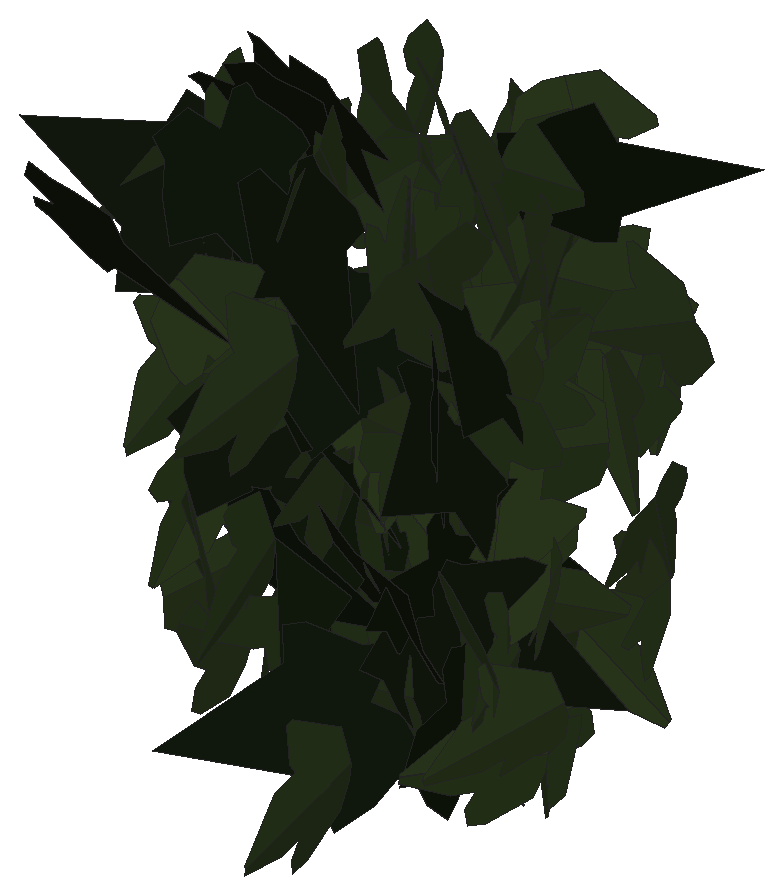
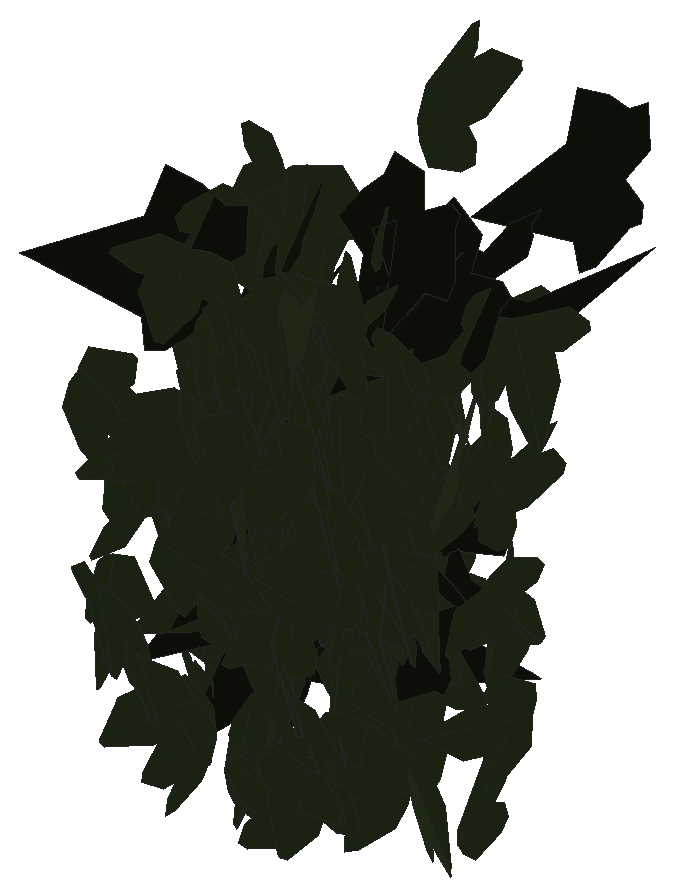
# SketchUp Ruby script. Lengths in inches.
U = 1.inch
M = Sketchup.active_model
def pt(a) = Geom::Point3d.new(a.map { |v| v * U })
def face(e, loops, mat)
  f = e.add_face(loops[0].map { |a| pt(a) })
  loops[1..].each { |l| e.add_face(l.map { |a| pt(a) }).erase! }
  f.material = f.back_material = mat if mat
  f
end
# faces: each face lists its corners as indices into pts; further lists are holes
def faces(e, pts, list, mat = nil) = list.each { |f| face(e, (f[0].is_a?(Array) ? f : [f]).map { |l| l.map { |i| pts[i] } }, mat) }
# xy, xz, yz: faces in a plane at the given z, y or x. An outline is a flat list of corners, or four numbers for a rectangle; further outlines are holes
def ring(l) = l.size == 4 ? [[l[0], l[1]], [l[2], l[1]], [l[2], l[3]], [l[0], l[3]]] : l.each_slice(2).to_a
def flat(e, list, mat, &to3) = list.each { |f| face(e, (f[0].is_a?(Array) ? f : [f]).map { |l| ring(l).map { |u, v| to3.(u, v) } }, mat) }
def xy(e, z, list, mat = nil) = flat(e, list, mat) { |x, y| [x, y, z] }
def xz(e, y, list, mat = nil) = flat(e, list, mat) { |x, z| [x, y, z] }
def yz(e, x, list, mat = nil) = flat(e, list, mat) { |y, z| [x, y, z] }
def lines(e, pts, list) = list.each { |a, b| e.add_line(pt(pts[a]), pt(pts[b])) }
# prism: a flat outline (further loops are holes) pulled along v
def prism(e, loops, v, mat = nil)
  f = face(e, loops, mat); d = Geom::Vector3d.new(v.map { |x| x * U })
  f.pushpull(f.normal.samedirection?(d) ? d.length : -d.length)
end
def box(e, o, s, mat = nil) = prism(e, [[o, [o[0] + s[0], o[1], o[2]], [o[0] + s[0], o[1] + s[1], o[2]], [o[0], o[1] + s[1], o[2]]]], [0, 0, s[2]], mat)
def at(x, y, z, deg = 0) = Geom::Transformation.translation(pt([x, y, z])) * Geom::Transformation.rotation(ORIGIN, Z_AXIS, deg.degrees)
def axes(o, x, y, z) = Geom::Transformation.new([*x, 0, *y, 0, *z, 0, *pt(o).to_a, 1])
def part(name) = M.definitions.add(name)
# library, detail: a bought-in or finely detailed component or shape, given as its bounding box
def library(name, o, s) = part(name).tap { |d| box(d.entities, o, s) }
def detail(e, o, s) = box(e.add_group.entities, o, s)
def put(e, d, t, mat = nil) = e.add_instance(d, t).tap { |i| i.material = mat if mat }
def group(e, t, mat = nil) = e.add_group.tap { |g| g.transformation = t; g.material = mat if mat }.entities
root = M.entities
M.materials.add("efeu1").color = [18, 25, 13]
M.materials.add("efeu2").color = [43, 57, 29]
c1 = part("ivyleaf_10")
p = [[0,0.5,-0.03],[-0.0625,2.02,-0.43],[-0.19,2.01,-0.46],[-0.54,1.05,-0.29],[-0.52,0.625,-0.18],[-0.83,0.76,-0.28],
  [-1.16,0.64,-0.33],[-1.15,0.33,-0.24],[-0.77,-0.39,0.02],[-0.3,-0.51,0.16],[0.04,-0.48,0.23],[-0.02,2.01,-0.4375],
  [-0.06,2.01,-0.43],[0.04,-0.49,0.23],[0.67,-0.49,0.14],[1.38,0.36,-0.2],[1.375,0.51,-0.24],[0.81,0.65,-0.19],
  [0.62,0.59,-0.15],[0.6,1.09,-0.28],[0.5,1.23,-0.31]]
faces(c1.entities,p,[[0,1,2,3,4,5,6,7,8,9,10],[11,12,0,13,14,15,16,17,18,19,20]],"efeu2")
c2 = part("ivyleaf_9")
p = [[1.54,2.16,1.25],[1.36,2.04,1.19],[-0.21,0.99,0.68],[-0.71,1.11,0.82],[-0.85,0.86,0.67],[-0.8,0.17,0.21],
  [-0.9,-0.01,0.1],[-0.67,-0.16,-0.02],[-0.08,-0.08,-0.05],[-0.03,-0.6,-0.4],[0.65,-0.88,-0.66],[0.83,-0.6,-0.49],
  [1.29,-0.42,-0.43],[1.8125,-0.07,-0.26],[1.21,0.44,0.15]]
faces(c2.entities,p,[[0,1,2,3,4,5,6,7,8,9,10,11,12,13,14]],"efeu1")
put(root,c1,axes([515.47,138.4375,160.84],[0.539,-0.35639,0.20084],[0.16726,-0.11118,-0.64617],[0.37332,0.56436,-0.00046]))
put(root,c1,axes([515.72,135.73,163.17],[-0.05856,-0.77801,0.02963],[-0.00282,-0.0295,-0.78021],[0.77857,-0.05862,-0.0006]))
put(root,c1,axes([515.53,136.83,156.8],[-0.18804,0.38277,0.56609],[0.25825,-0.50379,0.42643],[0.63268,0.31941,-0.00581]))
put(root,c1,axes([515.55,136.06,157.87],[0.01918,0.05739,-0.63411],[0.31724,0.54919,0.0593],[0.55205,-0.31759,-0.01205]))
put(root,c1,axes([515.91,135.9375,161.38],[0.0328,-0.04201,0.63628],[-0.321,0.54943,0.05282],[-0.55098,-0.32259,0.0071]))
put(root,c2,axes([516.15,135.63,162.83],[-0.18346,-0.71733,-0.2546],[-0.06618,-0.24587,0.74041],[-0.75829,0.19501,-0.00303]))
put(root,c1,axes([515.9,136.94,161.3],[-0.39721,0.56291,0.18241],[0.07955,-0.1669,0.68828],[0.58635,0.40397,0.03019]))
put(root,c1,axes([515.88,136.1875,163.31],[0.01451,-0.12903,-0.69764],[0.07537,0.69412,-0.12681],[0.70546,-0.0715,0.0279]))
put(root,c1,axes([515.82,137.53,157.49],[0.34018,-0.5829,0.20911],[0.1053,-0.18066,-0.6749],[0.61025,0.35611,-0.00012]))
put(root,c1,axes([516.02,135.91,159.39],[0.21441,0.45945,-0.40181],[-0.16104,-0.36821,-0.50696],[-0.58874,0.26804,-0.00766]))
put(root,c1,axes([515.92,135.77,160.82],[-0.21052,-0.17023,0.70196],[0.25805,-0.70064,-0.09252],[0.67464,0.21488,0.25443]))
put(root,c1,axes([515.99,138.02,157.55],[0.03211,-0.15718,0.61639],[0.02455,0.61702,0.15606],[-0.63564,0.01589,0.03717]))
put(root,c1,axes([516.1875,135.58,158.35],[-0.5527,0.37791,0.20592],[0.16367,-0.12541,0.66946],[0.39803,0.57632,0.01065]))
put(root,c1,axes([516.28,136.73,160.76],[-0.17633,0.40716,0.56258],[0.13587,-0.54899,0.43991],[0.68104,0.21494,0.05789]))
put(root,c1,axes([516.39,136.84,162.78],[-0.05447,-0.67467,0.07165],[-0.00268,-0.07167,-0.67685],[0.67846,-0.05445,0.00307]))
put(root,c1,axes([516.07,135.79,161.91],[-0.07922,0.03285,0.69201],[0.55018,-0.42031,0.08294],[0.42102,0.55543,0.02183]))
put(root,c1,axes([516.81,138.02,160.22],[0.08594,0.11931,0.62257],[-0.34551,-0.51792,0.14695],[0.53146,-0.356,-0.00514]))
put(root,c1,axes([516.66,137.69,159.83],[0.53776,-0.26423,-0.22129],[-0.18982,0.11524,-0.59889],[0.28768,0.56998,0.01849]))
put(root,c1,axes([516.1875,137.8,159.58],[0.20256,-0.20956,0.64495],[0.54856,-0.3451,-0.28442],[0.39869,0.58129,0.06365]))
put(root,c2,axes([516.22,136.1875,163.97],[0.7787,0.11175,0.06692],[0.06543,0.0152,-0.78665],[-0.11264,0.78142,0.00573]))
put(root,c1,axes([516.61,136.86,160.27],[-0.06321,-0.46032,-0.55569],[0.10713,0.54565,-0.46418],[0.71359,-0.12269,0.02047]))
put(root,c1,axes([516.73,138.66,158.58],[0.49284,-0.35342,-0.19578],[-0.16123,0.11112,-0.60645],[0.37046,0.51853,-0.00348]))
put(root,c1,axes([516.74,138.66,163.31],[0.4241,-0.45929,-0.17252],[-0.10901,0.13413,-0.62506],[0.47836,0.43776,0.01051]))
put(root,c1,axes([516.64,136.08,162.38],[0.40695,-0.44425,0.29438],[0.18072,-0.23341,-0.60207],[0.50135,0.44473,-0.02193]))
put(root,c2,axes([516.53,135.47,163.83],[0.25458,-0.63931,-0.38369],[-0.12098,0.36465,-0.68785],[0.73574,0.28117,0.01966]))
put(root,c1,axes([516.55,138.86,157.84],[0.59436,0.14862,0.25352],[0.24149,0.07893,-0.61243],[-0.16746,0.64133,0.01662]))
put(root,c1,axes([516.83,137.87,160.32],[0.08864,-0.31802,0.67164],[-0.07716,0.6688,0.32686],[-0.73911,-0.10796,0.04643]))
put(root,c1,axes([516.92,136.72,161.2],[-0.14642,-0.48517,0.45122],[0.05704,-0.46962,-0.48644],[0.6601,-0.06703,0.14212]))
put(root,c2,axes([516.29,133.05,163.9375],[0.68849,-0.2504,0.31362],[0.2994,-0.09424,-0.7325],[0.26725,0.75066,0.01266]))
put(root,c1,axes([517.02,138.37,161.9375],[-0.01516,0.10194,0.6291],[-0.25343,0.57642,-0.09951],[-0.58475,-0.25247,0.02682]))
put(root,c1,axes([516.83,135.89,158.97],[0.14306,-0.40908,0.65552],[0.20567,-0.62245,-0.43333],[0.74482,0.25045,-0.00625]))
put(root,c2,axes([516.6875,135.82,160.62],[0.0129,-0.40531,-0.66696],[0.04004,0.66651,-0.40426],[0.77942,-0.02753,0.03181]))
put(root,c1,axes([516.5,137.08,162.71],[0.16001,-0.0032,-0.62674],[0.62292,-0.07054,0.1594],[-0.06913,-0.64298,-0.01437]))
put(root,c1,axes([517.19,137.93,161.71],[0.37199,-0.51984,-0.35564],[-0.21389,0.28423,-0.63918],[0.59242,0.42904,-0.00746]))
put(root,c1,axes([516.75,137.95,157.75],[0.14098,0.07909,-0.65416],[0.41356,0.51018,0.15081],[0.51298,-0.43304,0.0582]))
put(root,c1,axes([517.12,135.98,158.04],[-0.55319,-0.3505,-0.07329],[0.06873,0.02845,-0.65476],[0.35143,-0.5573,0.01268]))
put(root,c1,axes([517.14,136.875,159.9375],[0.09685,-0.70342,0.15714],[0.01006,-0.15722,-0.70997],[0.72069,0.09673,-0.01121]))
put(root,c2,axes([517.01,136.07,164.48],[0.73513,0.05142,-0.30835],[-0.3079,-0.0172,-0.73691],[-0.05408,0.79699,0.00399]))
put(root,c1,axes([517.2,138.51,157.22],[0.1212,-0.47666,0.43195],[-0.07476,0.42614,0.49122],[-0.63891,-0.14029,0.02447]))
put(root,c1,axes([516.95,137.76,158.11],[0.2671,-0.27729,0.5144],[0.45029,-0.26284,-0.37549],[0.37248,0.51659,0.08506]))
put(root,c1,axes([517.34,136.73,157.66],[0.05018,-0.44885,0.47814],[0.02767,-0.47767,-0.4513],[0.65523,0.05454,-0.01756]))
put(root,c2,axes([516.6875,136.04,158.625],[0.34854,-0.25759,0.64088],[0.49786,-0.40389,-0.43309],[0.47877,0.60752,-0.0162]))
put(root,c1,axes([517.4375,136.98,158.77],[0.10026,-0.47514,-0.43178],[-0.055,0.42905,-0.4849],[0.63966,0.11136,0.02598]))
put(root,c1,axes([517.42,137.52,161.98],[0.09028,-0.14104,-0.66146],[-0.01055,0.66695,-0.14365],[0.67625,0.02923,0.08606]))
put(root,c1,axes([516.91,134.53,162.375],[0.32665,0.15414,0.55252],[0.50853,0.21635,-0.361],[-0.26538,0.60429,-0.01168]))
put(root,c1,axes([517.81,136.49,159.17],[-0.00404,0.02322,0.68184],[-0.5166,-0.44547,0.01211],[0.44561,-0.51622,0.02022]))
put(root,c1,axes([516.875,137.54,163.37],[0.01091,-0.01962,0.78333],[0.76375,-0.17483,-0.01501],[0.17513,0.76365,0.01669]))
put(root,c1,axes([517.42,138.01,159.39],[-0.09875,-0.07197,0.66743],[0.20307,-0.64621,-0.03964],[0.63985,0.19398,0.11559]))
put(root,c1,axes([517.59,135.76,163.85],[0.03427,-0.53437,-0.42188],[-0.02535,0.42112,-0.53546],[0.68036,0.0426,0.0013]))
put(root,c2,axes([517.58,136.18,159.7],[-0.66951,-0.24336,-0.3516],[0.33458,0.10861,-0.71228],[0.26627,-0.74838,0.01096]))
put(root,c1,axes([517.625,137.98,158.73],[0.46692,-0.55762,-0.06008],[-0.03546,0.04866,-0.72728],[0.55972,0.46825,0.00404]))
put(root,c1,axes([517.6875,136.81,161.93],[-0.23599,-0.6555,-0.03047],[0.00992,0.02881,-0.69668],[0.65613,-0.2362,-0.00043]))
put(root,c1,axes([517.29,136.88,162.77],[-0.41062,-0.26972,0.49443],[0.41315,0.27161,0.49128],[-0.38278,0.58249,-0.00013]))
put(root,c1,axes([517.69,135.3,161.5625],[-0.05989,0.22654,0.64254],[0.02986,-0.64352,0.22967],[0.68065,0.04816,0.04646]))
put(root,c2,axes([517.29,135.55,161.3125],[0.6265,-0.45291,-0.16641],[-0.12256,0.11441,-0.77279],[0.46669,0.63804,0.02045]))
put(root,c1,axes([517.98,137.35,160.51],[0.34204,-0.28019,-0.48652],[-0.37756,0.30684,-0.44215],[0.41552,0.50945,-0.00128]))
put(root,c1,axes([517.85,135.83,160.18],[-0.00176,-0.69906,-0.01878],[-0.00086,0.01878,-0.69906],[0.69931,-0.00174,-0.00091]))
put(root,c1,axes([517.43,138.03,163.17],[-0.19853,-0.02629,0.61256],[0.53481,-0.32229,0.1595],[0.29983,0.55747,0.1211]))
put(root,c1,axes([518.27,139.18,160.68],[0.24385,0.02609,-0.59989],[-0.59605,0.08886,-0.23842],[0.07265,0.64144,0.05743]))
put(root,c1,axes([517.68,135.98,161.21],[-0.11512,-0.43546,0.48275],[0.18888,0.44671,0.448],[-0.62209,0.21622,0.04669]))
put(root,c1,axes([518.09,136.86,162.35],[0.48523,-0.20979,0.38706],[-0.35689,0.14985,0.52863],[-0.25779,-0.60234,-0.0033]))
put(root,c1,axes([518.03,137.18,163.34],[-0.67099,-0.21035,0.00415],[-0.0033,-0.00333,-0.70318],[0.21037,-0.67099,0.00219]))
put(root,c2,axes([517.58,135.26,163.48],[-0.27511,-0.15245,-0.73315],[0.69016,0.25147,-0.31126],[0.29058,-0.74159,0.04517]))
put(root,c2,axes([518.46,135.39,157.7],[-0.11366,-0.23589,-0.72644],[-0.30415,-0.65972,0.26181],[-0.70061,0.32466,0.0042]))
put(root,c1,axes([518.05,138.4,161.82],[0.01785,0.25278,0.58916],[-0.09041,0.58449,-0.24804],[-0.63469,-0.07615,0.0519]))
put(root,c1,axes([518.1,136.45,158.7],[-0.54931,0.49453,0.16703],[0.11919,-0.11723,0.73909],[0.50818,0.56205,0.0072]))
put(root,c1,axes([518.33,135.72,159.67],[-0.19329,0.29154,0.5715],[-0.32061,0.47311,-0.34978],[-0.55571,-0.37436,0.00302]))
put(root,c1,axes([517.78,138.71,162.9375],[0.23797,-0.1003,0.60244],[0.56247,-0.21592,-0.25813],[0.23795,0.61069,0.00767]))
put(root,c1,axes([518.75,135.64,157.85],[-0.15452,0.03496,0.65248],[-0.65333,0.00265,-0.15486],[-0.01064,-0.67052,0.03341]))
put(root,c1,axes([518.09,136.79,159.23],[-0.3369,-0.36166,-0.53534],[0.41501,0.34156,-0.49192],[0.49512,-0.53238,0.04807]))
put(root,c1,axes([518.24,137.66,157.51],[-0.02701,0.02299,0.68133],[0.33188,-0.59516,0.03324],[0.59547,0.33275,0.01238]))
put(root,c1,axes([518.32,135.99,160.97],[0.60682,0.27232,0.03624],[0.03271,0.01563,-0.66513],[-0.27277,0.6077,0.00087]))
put(root,c1,axes([518.83,135.45,161.11],[0.25609,-0.21754,-0.58474],[-0.44784,0.37598,-0.33601],[0.43438,0.51588,-0.00169]))
put(root,c1,axes([518.82,138.46,160.41],[0.38761,-0.23797,-0.54593],[-0.44313,0.31993,-0.45408],[0.39788,0.58815,0.02612]))
put(root,c2,axes([518.09,135.42,162.09],[0.15296,-0.26991,-0.70732],[0.17711,0.71435,-0.23429],[0.73606,-0.1158,0.20336]))
put(root,c1,axes([518.52,137.34,157.24],[-0.51388,0.41527,0.00716],[-0.00565,0.0044,-0.6607],[-0.4153,-0.51391,0.00013]))
put(root,c1,axes([518.16,137.32,158.22],[-0.22289,0.22834,-0.63439],[0.46271,-0.43418,-0.31885],[-0.4904,-0.51344,-0.01251]))
put(root,c1,axes([518.66,137.8,161.16],[0.33154,-0.55712,-0.18708],[-0.09081,0.16365,-0.64829],[0.58063,0.34371,0.00543]))
put(root,c1,axes([518.52,137.21,161.96],[0.0409,0.65698,0.11134],[0.00129,0.11148,-0.65823],[-0.66635,0.04054,0.00556]))
put(root,c1,axes([518.68,138,163.0625],[0.10377,-0.6811,0.11836],[0.00631,-0.11875,-0.68887],[0.69128,0.10333,-0.01148]))
put(root,c1,axes([518.19,136.86,160.8],[0.18372,-0.1444,-0.69529],[0.60657,0.40536,0.07609],[0.36927,-0.59402,0.22094]))
put(root,c2,axes([518.28,135.89,158.63],[-0.15621,-0.22394,0.73655],[0.40678,-0.66208,-0.11503],[0.65359,0.35854,0.24763]))
put(root,c1,axes([518.76,136.82,160.83],[-0.23499,-0.64818,-0.11921],[0.03654,0.11355,-0.68945],[0.65804,-0.23777,-0.00429]))
put(root,c1,axes([518.93,135.31,162.8125],[-0.06414,0.37584,-0.55475],[-0.14356,0.53663,0.38017],[0.65451,0.15454,0.02902]))
put(root,c1,axes([518.93,137.09,156.35],[-0.60176,0.26805,-0.09464],[-0.09451,0.0203,0.65847],[0.2681,0.60882,0.01971]))
put(root,c1,axes([518.67,134.48,157.22],[0.01884,-0.12677,0.74134],[0.23223,-0.70435,-0.12635],[0.71535,0.232,0.0215]))
put(root,c1,axes([518.89,137.61,159.15],[-0.01423,-0.19416,0.63171],[0.04185,-0.63086,-0.19296],[0.65955,0.03584,0.02587]))
put(root,c1,axes([518.71,140.14,160.25],[0.60787,-0.18495,0.17352],[0.16407,-0.05682,-0.63535],[0.19337,0.62959,-0.00637]))
put(root,c1,axes([518.93,138.12,162.18],[0.15689,-0.42722,0.47587],[0.25555,-0.40727,-0.44989],[0.58623,0.29188,0.06877]))
put(root,c1,axes([519.21,137.73,156.97],[0.06705,-0.14594,0.67639],[-0.26681,0.62155,0.16056],[-0.63845,-0.27508,0.00394]))
put(root,c1,axes([519.42,136.31,158.74],[0.50469,0.32662,0.47915],[-0.40572,-0.25496,0.60114],[0.41432,-0.64753,0.00499]))
put(root,c1,axes([519.68,135.74,158.47],[-0.1714,0.2018,-0.7736],[-0.60636,0.48284,0.2603],[0.52107,0.62825,0.04844]))
put(root,c2,axes([519.16,135.74,159.54],[-0.05185,0.11828,-0.80072],[-0.25244,0.75998,0.12861],[0.76904,0.25744,-0.01177]))
put(root,c1,axes([519.55,137.55,160.27],[-0.0012,-0.03494,0.72083],[-0.35823,-0.62573,-0.03093],[0.6265,-0.35786,-0.0163]))
put(root,c2,axes([519.34,135.8,157.85],[0.00427,0.14639,-0.80813],[-0.44282,0.68102,0.12103],[0.69168,0.43509,0.08247]))
put(root,c2,axes([519.58,135.22,161.94],[0.22702,-0.07707,-0.74803],[-0.69685,0.27213,-0.23952],[0.28264,0.73282,0.01028]))
put(root,c1,axes([519.12,138.05,163.95],[0.54632,0.30182,0.21961],[0.18531,0.11861,-0.624],[-0.32401,0.57673,0.01341]))
put(root,c1,axes([519.1,138.3125,161.77],[-0.20908,-0.19712,-0.57341],[0.44522,0.36184,-0.28673],[0.41162,-0.49151,0.01888]))
put(root,c1,axes([518.98,137.32,162.86],[0.46232,-0.14543,0.57141],[0.54105,-0.18397,-0.48458],[0.23435,0.71162,-0.0085]))
put(root,c1,axes([519.39,136.69,161.47],[-0.04409,-0.74002,-0.05515],[0.01888,-0.05635,0.741],[-0.74183,0.04255,0.02214]))
put(root,c1,axes([519.5625,135.11,163.42],[-0.2058,-0.72629,-0.2237],[0.04999,0.21832,-0.75481],[0.75831,-0.2115,-0.01095]))
put(root,c1,axes([519.43,136.4375,159.69],[0.53628,0.35861,-0.08298],[0.06363,0.05411,0.64506],[0.36254,-0.53996,0.00954]))
put(root,c2,axes([519.17,135.85,158.77],[0.06206,-0.06809,-0.79572],[0.11843,0.79008,-0.05837],[0.7898,-0.11312,0.07128]))
put(root,c1,axes([519.19,136.6875,158.29],[0.41324,-0.26035,0.47838],[0.42555,-0.22041,-0.48756],[0.3399,0.59248,0.02883]))
put(root,c1,axes([519.41,136.8125,163.88],[-0.19805,-0.34664,-0.54634],[0.25925,0.48099,-0.39915],[0.59283,-0.32614,-0.00797]))
put(root,c1,axes([519.74,135.71,161.49],[-0.69086,-0.41606,0.1363],[-0.11517,-0.07295,-0.80646],[0.4224,-0.70039,0.00303]))
put(root,c1,axes([519.24,136.24,164.24],[-0.33719,0.34555,-0.56953],[0.41384,-0.39157,-0.48258],[-0.52203,-0.53361,-0.01469]))
put(root,c1,axes([519.36,136.82,161.25],[-0.51905,-0.24058,0.41209],[0.37298,0.17523,0.57209],[-0.29763,0.63916,-0.00173]))
put(root,c1,axes([519.62,136.65,162.01],[-0.1336,-0.27145,0.64108],[0.14148,-0.64974,-0.24563],[0.68165,0.08165,0.17663]))
put(root,c1,axes([519.22,138.08,157.68],[0.35013,0.14014,0.53567],[0.48609,0.22568,-0.37677],[-0.26513,0.59883,0.01663]))
put(root,c1,axes([519.68,138.24,160.39],[0.11496,0.52621,-0.39602],[0.0761,0.3887,0.53858],[0.65417,-0.13769,0.00694]))
put(root,c1,axes([519.46,136.5625,158.93],[-0.21743,-0.25233,-0.66481],[0.42787,0.50883,-0.33307],[0.56795,-0.47994,-0.00359]))
put(root,c1,axes([519.62,132.33,163.43],[-0.0584,-0.03435,0.82545],[0.23863,-0.79293,-0.01611],[0.79095,0.2367,0.06581]))
put(root,c1,axes([519.98,136.69,156.79],[0.41841,-0.23437,0.49683],[-0.44258,0.22615,0.4794],[-0.32542,-0.60891,-0.01319]))
put(root,c1,axes([519.94,136.11,157.27],[-0.02996,0.08809,0.64845],[-0.14958,-0.63287,0.07906],[0.63709,-0.14445,0.04906]))
put(root,c1,axes([519.63,136.58,158.36],[-0.01272,-0.16958,0.62032],[0.29499,-0.55285,-0.14509],[0.57143,0.28163,0.0887]))
put(root,c1,axes([519.95,136.63,159.25],[0.38995,-0.44132,-0.24467],[-0.16348,0.18204,-0.58891],[0.47738,0.42283,-0.00182]))
put(root,c1,axes([520.15,138.13,158.5],[0.38938,-0.32591,-0.41907],[-0.33029,0.25817,-0.50765],[0.41563,0.51047,-0.01081]))
put(root,c2,axes([519.66,135.51,161.39],[0.3505,-0.35539,-0.59071],[0.39311,-0.44134,0.49877],[-0.56631,-0.52632,-0.01937]))
put(root,c2,axes([519.38,137.37,163.45],[0.37846,0.06599,0.67345],[0.66101,0.12905,-0.38411],[-0.14479,0.76165,0.00673]))
put(root,c1,axes([520.4375,138.21,161.78],[-0.26872,-0.04017,0.6118],[-0.59894,-0.12561,-0.27132],[0.13108,-0.6563,0.01448]))
put(root,c1,axes([520.01,138.36,159.28],[0.02492,-0.57452,-0.28179],[0.01687,0.28249,-0.57446],[0.63968,0.01493,0.02613]))
put(root,c1,axes([520.15,136.15,157.82],[-0.04641,-0.2146,0.61928],[-0.14827,-0.60129,-0.21948],[0.63841,-0.15525,-0.00596]))
put(root,c1,axes([519.67,137.97,160.81],[0.47655,-0.15382,0.43059],[0.42778,-0.06963,-0.49831],[0.16146,0.63848,0.04939]))
put(root,c2,axes([519.7,135.74,162.41],[0.00583,-0.47755,0.6402],[0.17701,-0.62352,-0.46672],[0.77883,0.14529,0.10128]))
